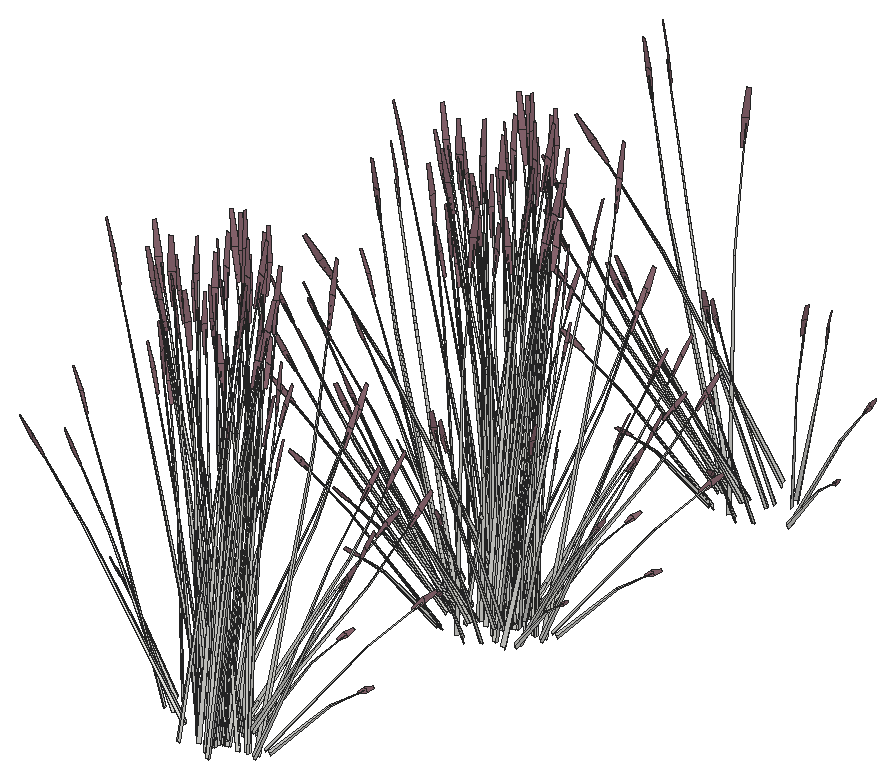
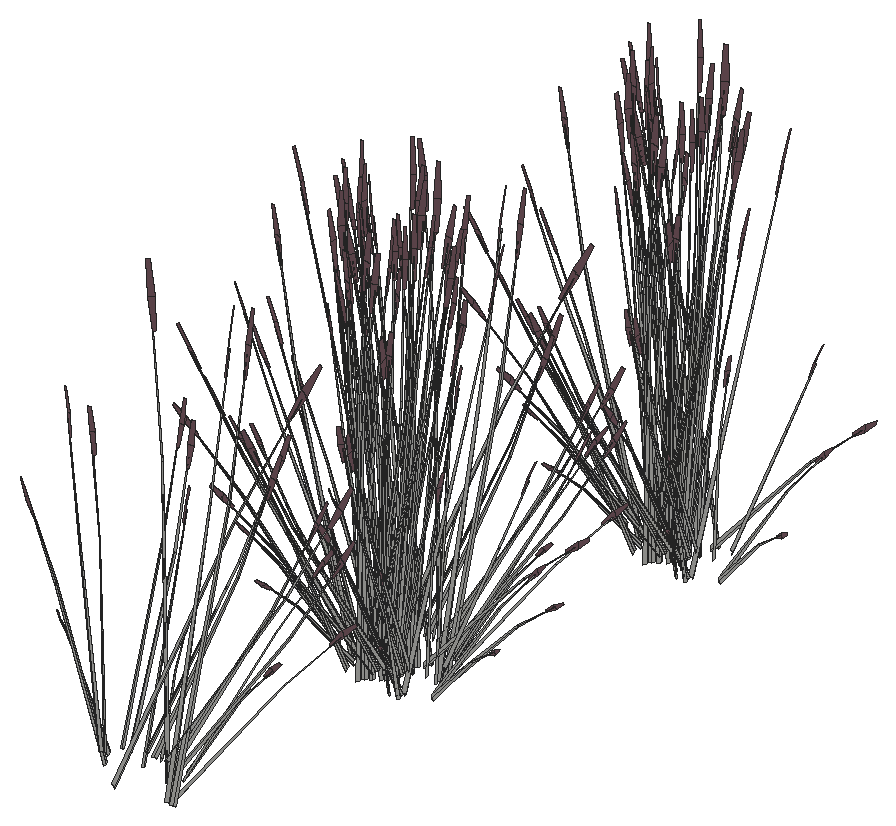
# SketchUp Ruby script. Lengths in inches.
U = 1.inch
M = Sketchup.active_model
def pt(a) = Geom::Point3d.new(a.map { |v| v * U })
def face(e, loops, mat)
  f = e.add_face(loops[0].map { |a| pt(a) })
  loops[1..].each { |l| e.add_face(l.map { |a| pt(a) }).erase! }
  f.material = f.back_material = mat if mat
  f
end
# faces: each face lists its corners as indices into pts; further lists are holes
def faces(e, pts, list, mat = nil) = list.each { |f| face(e, (f[0].is_a?(Array) ? f : [f]).map { |l| l.map { |i| pts[i] } }, mat) }
# xy, xz, yz: faces in a plane at the given z, y or x. An outline is a flat list of corners, or four numbers for a rectangle; further outlines are holes
def ring(l) = l.size == 4 ? [[l[0], l[1]], [l[2], l[1]], [l[2], l[3]], [l[0], l[3]]] : l.each_slice(2).to_a
def flat(e, list, mat, &to3) = list.each { |f| face(e, (f[0].is_a?(Array) ? f : [f]).map { |l| ring(l).map { |u, v| to3.(u, v) } }, mat) }
def xy(e, z, list, mat = nil) = flat(e, list, mat) { |x, y| [x, y, z] }
def xz(e, y, list, mat = nil) = flat(e, list, mat) { |x, z| [x, y, z] }
def yz(e, x, list, mat = nil) = flat(e, list, mat) { |y, z| [x, y, z] }
def lines(e, pts, list) = list.each { |a, b| e.add_line(pt(pts[a]), pt(pts[b])) }
# prism: a flat outline (further loops are holes) pulled along v
def prism(e, loops, v, mat = nil)
  f = face(e, loops, mat); d = Geom::Vector3d.new(v.map { |x| x * U })
  f.pushpull(f.normal.samedirection?(d) ? d.length : -d.length)
end
def box(e, o, s, mat = nil) = prism(e, [[o, [o[0] + s[0], o[1], o[2]], [o[0] + s[0], o[1] + s[1], o[2]], [o[0], o[1] + s[1], o[2]]]], [0, 0, s[2]], mat)
def at(x, y, z, deg = 0) = Geom::Transformation.translation(pt([x, y, z])) * Geom::Transformation.rotation(ORIGIN, Z_AXIS, deg.degrees)
def axes(o, x, y, z) = Geom::Transformation.new([*x, 0, *y, 0, *z, 0, *pt(o).to_a, 1])
def part(name) = M.definitions.add(name)
# library, detail: a bought-in or finely detailed component or shape, given as its bounding box
def library(name, o, s) = part(name).tap { |d| box(d.entities, o, s) }
def detail(e, o, s) = box(e.add_group.entities, o, s)
def put(e, d, t, mat = nil) = e.add_instance(d, t).tap { |i| i.material = mat if mat }
def group(e, t, mat = nil) = e.add_group.tap { |g| g.transformation = t; g.material = mat if mat }.entities
root = M.entities
M.materials.add("LightPink_Translucent").color = [144, 107, 117]
c1 = part("blade")
p = [[2.15,0.21,22],[0,0.17,0],[0.09,0.45,0],[2.18,0.31,22],[2.29,0.31,22],[0.38,0.45,0],
  [2.48,0.24,33],[2.49,0.24,33],[2.48,0.22,33]]
faces(c1.entities,p,[[0,1,2,3],[4,5,2,3],[6,3,4,7],[8,0,3,6]])
c2 = part("seeds")
p = [[0.3,-0.1,1.38],[-0.01,-0.03,1.59],[-0.01,-0.03,0.03],[0.14,-0.07,-0.07],[0.29,-0.03,3],[0.15,0.01,3.11]]
faces(c2.entities,p,[[0,1,2,3],[1,0,4,5]],"LightPink_Translucent")
c3 = part("blade with seeds")
put(c3.entities,c1,at(0,0,0))
put(c3.entities,c2,axes([2.4,0.25,30.99],[1.5799,-0.05474,1.17369],[-0.12525,1.92788,0.29478],[-0.07173,-0.02425,1.56792]))
put(root,c3,axes([33.5,392.59,44.36],[0.53281,1.15808,0.45755],[-1.52239,0.4027,0.17955],[0.01861,-0.2128,1.58856]))
put(root,c3,axes([40.95,393.48,43.98],[-0.7893,0.12429,1.41583],[-0.12563,-0.9893,0.08104],[0.55282,-0.14974,0.80566]))
put(root,c3,axes([33.24,393.5,44.72],[-0.59459,0.93321,0.44739],[-1.23546,-0.44912,-0.21531],[0,-0.21512,1.43643]))
put(root,c3,axes([35.42,392.69,44.21],[0,-1.19833,0],[1.53239,0,0],[0,0,1.79456]))
put(root,c3,axes([37.28,389.92,44.48],[-1.14694,-0.51783,0.49651],[0.68554,-0.92854,0],[0.26122,0.11794,1.57504]))
put(root,c3,axes([39.52,393.56,46.98],[1.07686,-0.45739,-0.71045],[0.60013,0.94154,0.08574],[0.52031,-0.10696,1.00501]))
put(root,c3,axes([34.69,391.93,44.36],[-1.01611,0.93987,0.45755],[-1.20717,-0.82966,0.17955],[0.24496,-0.0938,1.58856]))
put(root,c3,axes([35.8,393.62,44.3],[-1.1399,-0.8914,-0.06131],[1.1406,-0.89194,0],[-0.03981,-0.03113,1.75571]))
put(root,c3,axes([32.93,390.39,44.47],[-0.35402,1.02926,0.17642],[-1.29548,-0.29127,0.35086],[0.22379,-0.00501,1.60407]))
put(root,c3,axes([35.64,391.53,44.62],[0.23642,-0.92427,0.1448],[1.15506,0.16044,-0.41347],[0.21021,0.09491,1.26744]))
put(root,c3,axes([33.64,393.73,44.36],[1.54892,0.2182,0.45755],[-0.31522,1.23236,0.17955],[-0.22636,-0.119,1.58856]))
put(root,c3,axes([35.14,391.77,44.72],[-0.73619,-0.86927,0.44739],[1.11511,-0.61213,-0.21531],[0.23824,0.10756,1.43643]))
put(root,c3,axes([32.8,395.7,44.47],[1.31687,-0.27488,0.17642],[0.32517,1.02297,0.35086],[-0.11745,-0.14905,1.60407]))
put(root,c3,axes([36.46,392.96,44.21],[1.37109,0,0],[0,1.07219,0],[0,0,1.78407]))
put(root,c3,axes([36.85,390.44,44.47],[-1.31687,0.27488,0.17642],[-0.32517,-1.02297,0.35086],[0.11745,0.14905,1.60407]))
put(root,c3,axes([36.02,392.41,44.38],[-1.54892,-0.2182,0.49198],[0.31522,-1.23236,0.19306],[0.22636,0.119,1.70813]))
put(root,c3,axes([34.78,395.45,44.2],[-0.39985,-0.89288,0],[1.1418,-0.31268,0],[0,0,1.54371]))
put(root,c3,axes([34.02,394.61,44.62],[-0.23642,0.92427,0.1448],[-1.15506,-0.16044,-0.41347],[-0.21021,-0.09491,1.26744]))
put(root,c3,axes([36.72,395.75,44.47],[0.35402,-1.02926,0.17642],[1.29548,0.29127,0.35086],[-0.22379,0.00501,1.60407]))
put(root,c3,axes([36.43,393.42,44.21],[0.85545,0.66896,0],[-0.85545,0.66896,0],[0,0,1.69266]))
put(root,c3,axes([31.57,392.16,45.34],[0.34834,-0.14982,1.77064],[0.12012,1.04605,0.13857],[-0.75452,0.1388,0.63284]))
put(root,c3,axes([38.75,393.125,44.47],[-0.96285,-0.75439,0.17642],[0.97031,-0.7317,0.35086],[-0.10634,0.15406,1.60407]))
put(root,c3,axes([42.6,393.82,44.77],[-0.75718,0.17097,1.1486],[0.35641,-0.70661,0.84392],[0.40168,0.04835,0.25299]))
put(root,c3,axes([34.5,395.86,44.2],[-1.23546,-0.46496,0],[0.59459,-0.96613,0],[0,0,1.62707]))
put(root,c3,axes([32.375,396.22,44.48],[1.14694,0.51783,0.49651],[-0.68554,0.92854,0],[-0.26122,-0.11794,1.57504]))
put(root,c3,axes([36.42,392.63,44.72],[0.59459,-0.93321,0.44739],[1.23546,0.44912,-0.21531],[0,0.21512,1.43643]))
put(root,c3,axes([36.19,393.17,44.29],[0,1.19774,-0.05637],[-1.53239,0,0],[0,0.03764,1.79368]))
put(root,c3,axes([29.16,392.73,46.68],[-0.332,0.94205,-0.51099],[-1.13828,-0.3229,-0.3958],[-0.45829,0.08638,0.97773]))
put(root,c3,axes([31.72,396.76,44.375],[-0.7662,1.03778,0],[-1.28187,-0.57875,-0.51607],[-0.29196,-0.13181,1.63711]))
put(root,c3,axes([39.54,393.15,44.48],[0,-1.03566,0.49651],[1.37109,0,0],[0,0.23588,1.57504]))
put(root,c3,axes([36.1,393.93,44.72],[1.33077,-0.06393,0.44739],[0.12035,1.06125,-0.21531],[-0.23824,0.10756,1.43643]))
put(root,c3,axes([36.93,392.85,44.62],[1.1418,-0.30203,0.1448],[0.39985,0.86246,-0.41347],[0,0.18981,1.26744]))
put(root,c3,axes([41.18,394.95,44.59],[-0.29514,-0.25472,1.43002],[0.38401,-0.84262,-0.30754],[0.59714,0.11414,0.61141]))
put(root,c3,axes([35.9,395.875,44.2],[1.23546,0.46496,0],[-0.59459,0.96613,0],[0,0,1.74954]))
put(root,c3,axes([36.39,396.9,44.19],[-0.75665,-1.04141,-0.05142],[1.28187,-0.57875,0.51607],[-0.31588,0.09915,1.6363]))
put(root,c3,axes([36.125,394.39,44.62],[0.90538,0.62224,0.1448],[-0.75521,0.70202,-0.41347],[-0.21021,0.09491,1.26744]))
put(root,c3,axes([38.47,395.46,46.98],[1.22504,0.02494,-0.71045],[-0.08228,1.05005,0.08574],[0.51899,0.11081,1.00501]))
put(root,c3,axes([37.09,396.3,44.48],[1.14694,-0.51783,0.49651],[0.68554,0.92854,0],[-0.26122,0.11794,1.57504]))
put(root,c3,axes([35.46,395.49,44.29],[0.53281,1.18979,-0.06012],[-1.52239,0.41691,0],[0.01861,0.04155,1.72173]))
put(root,c3,axes([27.8,394.94,44.59],[0.42589,0.08502,1.43002],[0.2745,0.86839,-0.30754],[-0.57851,0.16255,0.61141]))
put(root,c3,axes([40.47,393.33,44.375],[1.53239,0,0],[0,1.1575,-0.51607],[0,0.26363,1.63711]))
put(root,c3,axes([39.86,393.93,44.2],[-1.53164,-0.00828,-0.04976],[0,-1.1575,0.49943],[-0.04813,0.2635,1.58352]))
put(root,c3,axes([26.91,396.76,44.77],[0.51072,-0.46938,1.1486],[0.20153,0.74307,0.84392],[-0.36908,0.13305,0.25299]))
put(root,c3,axes([36.43,396.37,44.33],[1.53422,0.33662,0.30756],[-0.38383,1.20322,-0.36492],[-0.25393,0.15059,1.64885]))
put(root,c3,axes([38.39,396.26,44.77],[-0.69001,-0.29779,1.1486],[0.89096,-0.30257,0.84392],[0.24031,0.2563,0.25299]))
put(root,c3,axes([29.72,394.83,46.68],[0.31482,0.94565,-0.51099],[-1.19224,0.16542,-0.3958],[-0.34166,0.254,0.97773]))
put(root,c3,axes([37.36,397.02,44.375],[0.7662,1.03778,0],[-1.28187,0.57875,-0.51607],[-0.29196,0.13181,1.63711]))
put(root,c3,axes([36.71,392.91,44.84],[-0.03348,-0.97511,1.41272],[1.51511,0.25277,0.59816],[-0.35835,0.53357,1.3335]))
put(root,c3,axes([36.83,396.67,46.68],[1.20928,-0.24619,-0.51099],[0.21154,0.93233,-0.3958],[0.32481,0.26718,0.97773]))
put(root,c3,axes([38.5,397.62,44.67],[-0.78586,-0.03248,1.0506],[0.51898,-0.68985,0.58006],[0.31045,0.24509,0.8241]))
put(root,c3,axes([35.93,395.95,44.59],[0.02163,-0.34331,1.43002],[1.03345,-0.38348,-0.30754],[0.31903,0.4109,0.61141]))
put(root,c3,axes([31.24,398.81,44.77],[-0.03171,-0.6158,1.1486],[0.7925,0.43922,0.84392],[-0.15586,0.29352,0.25299]))
put(root,c3,axes([31.54,396.43,47],[0.87728,0.69587,-0.5672],[-0.92674,0.60943,-0.43934],[-0.13348,0.35356,1.08528]))
put(root,c3,axes([30.59,397.48,44.82],[1.11329,-0.1834,0.06507],[0.25594,0.73887,-0.86304],[-0.07058,0.37403,0.7736]))
put(root,c3,axes([34.14,397.11,46.68],[1.20468,0.25962,-0.51099],[-0.41292,0.89013,-0.3958],[0.11046,0.35838,0.97773]))
put(root,c3,axes([31.27,396.11,47.34],[-0.03189,0.95798,-0.7886],[-1.34277,-0.06434,0.09517],[-0.14171,0.40585,1.11556]))
put(root,c3,axes([33.7,396.9375,46.98],[0.5849,0.8421,-0.71045],[-1.20401,0.4693,0.08574],[0.13677,0.40688,1.00501]))
put(root,c3,axes([30.32,398.26,44.59],[0.38672,-0.16338,1.43002],[0.95481,0.49262,-0.30754],[-0.28419,0.42626,0.61141]))
put(root,c3,axes([30.82,397.46,45.36],[0.02693,-0.53464,1.54345],[1.21102,0.2824,0.21329],[-0.10493,0.5698,0.72882]))
put(root,c3,axes([44.9375,427.97,44.59],[-0.34835,0.20963,1.43002],[-1.04325,-0.36691,-0.30754],[0.19338,-0.4563,0.61141]))
put(root,c3,axes([43.35,428.7,46.98],[-0.5849,-0.8421,-0.71045],[1.20401,-0.4693,0.08574],[-0.13677,-0.40688,1.00501]))
put(root,c3,axes([39.55,427.57,44.59],[-0.07421,0.33879,1.43002],[-1.08488,0.28361,-0.30754],[-0.25359,-0.4379,0.61141]))
put(root,c3,axes([45.79,429.52,46.98],[0.03189,-0.95798,-0.71045],[1.34277,0.06434,0.08574],[0.14171,-0.40585,1.00501]))
put(root,c3,axes([42.91,428.53,46.68],[-1.20468,-0.25962,-0.51099],[0.41292,-0.89013,-0.3958],[-0.11046,-0.35838,0.97773]))
put(root,c3,axes([43.66,426.3,44.77],[0.15721,0.60392,1.1486],[-0.87211,-0.33448,0.84392],[0.09385,-0.30923,0.25299]))
put(root,c3,axes([45.51,429.2,46.68],[-0.87728,-0.69587,-0.51099],[0.92674,-0.60943,-0.3958],[0.13348,-0.35356,0.97773]))
put(root,c3,axes([39.17,427.03,44.77],[0.63926,0.36046,1.1486],[-0.93099,0.21668,0.84392],[-0.1992,-0.27702,0.25299]))
put(root,c3,axes([40.72,428.9375,46.98],[-1.04497,-0.50058,-0.71045],[0.74264,-0.8772,0.08574],[-0.3786,-0.29889,1.00501]))
put(root,c3,axes([40.23,428.96,46.68],[-1.20928,0.24619,-0.51099],[-0.21154,-0.93233,-0.3958],[-0.32481,-0.26718,0.97773]))
put(root,c3,axes([47.37,431.1875,46.98],[0.64013,-0.81717,-0.71045],[1.12174,0.58074,0.08574],[0.38221,-0.29607,1.00501]))
put(root,c3,axes([40.45,428.81,44.375],[-0.7662,-1.03778,0],[1.28187,-0.57875,-0.51607],[0.29196,-0.13181,1.63711]))
put(root,c3,axes([47.34,430.81,46.68],[-0.31482,-0.94565,-0.51099],[1.19224,-0.16542,-0.3958],[0.34166,-0.254,0.97773]))
put(root,c3,axes([43.22,434.6,45.33],[1.05902,0.41762,1.51261],[-1.03748,0.89969,0.59816],[-0.46471,-0.53324,1.26806]))
put(root,c3,axes([48.3,430.4375,44.59],[-0.4378,-0.03068,1.43002],[-0.44851,-0.8229,-0.30754],[0.53783,-0.23279,0.61141]))
put(root,c3,axes([48.8,428.93,44.77],[-0.40819,0.5272,1.1486],[-0.35086,-0.70831,0.84392],[0.33713,-0.17749,0.25299]))
put(root,c3,axes([37.34,432.5,44.375],[-1.53239,0,0],[0,-1.1575,-0.51607],[0,-0.26363,1.63711]))
put(root,c3,axes([37.6,430.43,44.59],[0.23927,0.28834,1.43002],[-0.55135,0.78376,-0.30754],[-0.56612,-0.18733,0.61141]))
put(root,c3,axes([38.59,430.18,46.98],[-1.22504,-0.02494,-0.71045],[0.08228,-1.05005,0.08574],[-0.51899,-0.11081,1.00501]))
put(root,c3,axes([38.52,432.19,44.33],[-1.1399,0.87071,0.30756],[-1.1406,-0.86155,-0.36492],[-0.03981,-0.24727,1.64885]))
put(root,c3,axes([42.15,432.6,44.43],[1.3808,0.50196,0.24065],[-0.66454,1.04299,0.50002],[0,-0.24043,1.60543]))
put(root,c3,axes([38.18,430.39,46.68],[-0.88986,0.68603,-0.51099],[-0.77932,-0.72471,-0.3958],[-0.45212,-0.10438,0.97773]))
put(root,c3,axes([36.17,431.3,44.77],[0.78239,-0.07411,1.1486],[-0.49629,0.65296,0.84392],[-0.38663,-0.09795,0.25299]))
put(root,c3,axes([41.7,431.9,44.72],[-1.33077,0.06393,0.44739],[-0.12035,-1.06125,-0.21531],[0.23824,-0.10756,1.43643]))
put(root,c3,axes([38.27,432.68,44.48],[0,1.03566,0.49651],[-1.37109,0,0],[0,-0.23588,1.57504]))
put(root,c3,axes([47.89,432.91,46.68],[0.332,-0.94205,-0.51099],[1.13828,0.3229,-0.3958],[0.45829,-0.08638,0.97773]))
put(root,c3,axes([46.09,429.07,44.375],[0.7662,-1.03778,0],[1.28187,0.57875,-0.51607],[0.29196,0.13181,1.63711]))
put(root,c3,axes([41.66,432.28,44.36],[0.53281,1.15808,0.45755],[-1.52239,0.4027,0.17955],[0.01861,-0.2128,1.58856]))
put(root,c3,axes([49.11,433.17,43.98],[-0.7893,0.12429,1.41583],[-0.12563,-0.9893,0.08104],[0.55282,-0.14974,0.80566]))
put(root,c3,axes([41.39,433.2,44.72],[-0.59459,0.93321,0.44739],[-1.23546,-0.44912,-0.21531],[0,-0.21512,1.43643]))
put(root,c3,axes([43.57,432.38,44.21],[0,-1.19833,0],[1.53239,0,0],[0,0,1.79456]))
put(root,c3,axes([45.43,429.61,44.48],[-1.14694,-0.51783,0.49651],[0.68554,-0.92854,0],[0.26122,0.11794,1.57504]))
put(root,c3,axes([47.67,433.25,46.98],[1.07686,-0.45739,-0.71045],[0.60013,0.94154,0.08574],[0.52031,-0.10696,1.00501]))
put(root,c3,axes([42.85,431.625,44.36],[-1.01611,0.93987,0.45755],[-1.20717,-0.82966,0.17955],[0.24496,-0.0938,1.58856]))
put(root,c3,axes([43.96,433.31,44.3],[-1.1399,-0.8914,-0.06131],[1.1406,-0.89194,0],[-0.03981,-0.03113,1.75571]))
put(root,c3,axes([41.08,430.08,44.47],[-0.35402,1.02926,0.17642],[-1.29548,-0.29127,0.35086],[0.22379,-0.00501,1.60407]))
put(root,c3,axes([43.79,431.22,44.62],[0.23642,-0.92427,0.1448],[1.15506,0.16044,-0.41347],[0.21021,0.09491,1.26744]))
put(root,c3,axes([41.79,433.42,44.36],[1.54892,0.2182,0.45755],[-0.31522,1.23236,0.17955],[-0.22636,-0.119,1.58856]))
put(root,c3,axes([43.29,431.47,44.72],[-0.73619,-0.86927,0.44739],[1.11511,-0.61213,-0.21531],[0.23824,0.10756,1.43643]))
put(root,c3,axes([40.96,435.39,44.47],[1.31687,-0.27488,0.17642],[0.32517,1.02297,0.35086],[-0.11745,-0.14905,1.60407]))
put(root,c3,axes([44.61,432.65,44.21],[1.37109,0,0],[0,1.07219,0],[0,0,1.78407]))
put(root,c3,axes([45,430.14,44.47],[-1.31687,0.27488,0.17642],[-0.32517,-1.02297,0.35086],[0.11745,0.14905,1.60407]))
put(root,c3,axes([44.17,432.1,44.38],[-1.54892,-0.2182,0.49198],[0.31522,-1.23236,0.19306],[0.22636,0.119,1.70813]))
put(root,c3,axes([42.93,435.15,44.2],[-0.39985,-0.89288,0],[1.1418,-0.31268,0],[0,0,1.54371]))
put(root,c3,axes([42.17,434.3,44.62],[-0.23642,0.92427,0.1448],[-1.15506,-0.16044,-0.41347],[-0.21021,-0.09491,1.26744]))
put(root,c3,axes([44.875,435.44,44.47],[0.35402,-1.02926,0.17642],[1.29548,0.29127,0.35086],[-0.22379,0.00501,1.60407]))
put(root,c3,axes([44.58,433.11,44.21],[0.85545,0.66896,0],[-0.85545,0.66896,0],[0,0,1.69266]))
put(root,c3,axes([39.72,431.85,45.34],[0.34834,-0.14982,1.77064],[0.12012,1.04605,0.13857],[-0.75452,0.1388,0.63284]))
put(root,c3,axes([46.9,432.82,44.47],[-0.96285,-0.75439,0.17642],[0.97031,-0.7317,0.35086],[-0.10634,0.15406,1.60407]))
put(root,c3,axes([50.75,433.51,44.77],[-0.75718,0.17097,1.1486],[0.35641,-0.70661,0.84392],[0.40168,0.04835,0.25299]))
put(root,c3,axes([42.65,435.55,44.2],[-1.23546,-0.46496,0],[0.59459,-0.96613,0],[0,0,1.62707]))
put(root,c3,axes([40.53,435.91,44.48],[1.14694,0.51783,0.49651],[-0.68554,0.92854,0],[-0.26122,-0.11794,1.57504]))
put(root,c3,axes([44.57,432.33,44.72],[0.59459,-0.93321,0.44739],[1.23546,0.44912,-0.21531],[0,0.21512,1.43643]))
put(root,c3,axes([44.34,432.86,44.29],[0,1.19774,-0.05637],[-1.53239,0,0],[0,0.03764,1.79368]))
put(root,c3,axes([37.32,432.42,46.68],[-0.332,0.94205,-0.51099],[-1.13828,-0.3229,-0.3958],[-0.45829,0.08638,0.97773]))
put(root,c3,axes([39.87,436.45,44.375],[-0.7662,1.03778,0],[-1.28187,-0.57875,-0.51607],[-0.29196,-0.13181,1.63711]))
put(root,c3,axes([47.69,432.85,44.48],[0,-1.03566,0.49651],[1.37109,0,0],[0,0.23588,1.57504]))
put(root,c3,axes([44.26,433.62,44.72],[1.33077,-0.06393,0.44739],[0.12035,1.06125,-0.21531],[-0.23824,0.10756,1.43643]))
put(root,c3,axes([45.09,432.54,44.62],[1.1418,-0.30203,0.1448],[0.39985,0.86246,-0.41347],[0,0.18981,1.26744]))
put(root,c3,axes([49.33,434.64,44.59],[-0.29514,-0.25472,1.43002],[0.38401,-0.84262,-0.30754],[0.59714,0.11414,0.61141]))
put(root,c3,axes([44.05,435.57,44.2],[1.23546,0.46496,0],[-0.59459,0.96613,0],[0,0,1.74954]))
put(root,c3,axes([44.55,436.6,44.19],[-0.75665,-1.04141,-0.05142],[1.28187,-0.57875,0.51607],[-0.31588,0.09915,1.6363]))
put(root,c3,axes([44.28,434.08,44.62],[0.90538,0.62224,0.1448],[-0.75521,0.70202,-0.41347],[-0.21021,0.09491,1.26744]))
put(root,c3,axes([46.62,435.15,46.98],[1.22504,0.02494,-0.71045],[-0.08228,1.05005,0.08574],[0.51899,0.11081,1.00501]))
put(root,c3,axes([45.24,436,44.48],[1.14694,-0.51783,0.49651],[0.68554,0.92854,0],[-0.26122,0.11794,1.57504]))
put(root,c3,axes([43.61,435.18,44.29],[0.53281,1.18979,-0.06012],[-1.52239,0.41691,0],[0.01861,0.04155,1.72173]))
put(root,c3,axes([35.95,434.63,44.59],[0.42589,0.08502,1.43002],[0.2745,0.86839,-0.30754],[-0.57851,0.16255,0.61141]))
put(root,c3,axes([48.62,433.02,44.375],[1.53239,0,0],[0,1.1575,-0.51607],[0,0.26363,1.63711]))
put(root,c3,axes([48.01,433.62,44.2],[-1.53164,-0.00828,-0.04976],[0,-1.1575,0.49943],[-0.04813,0.2635,1.58352]))
put(root,c3,axes([35.0625,436.45,44.77],[0.51072,-0.46938,1.1486],[0.20153,0.74307,0.84392],[-0.36908,0.13305,0.25299]))
put(root,c3,axes([44.58,436.0625,44.33],[1.53422,0.33662,0.30756],[-0.38383,1.20322,-0.36492],[-0.25393,0.15059,1.64885]))
put(root,c3,axes([46.54,435.96,44.77],[-0.69001,-0.29779,1.1486],[0.89096,-0.30257,0.84392],[0.24031,0.2563,0.25299]))
put(root,c3,axes([37.87,434.52,46.68],[0.31482,0.94565,-0.51099],[-1.19224,0.16542,-0.3958],[-0.34166,0.254,0.97773]))
put(root,c3,axes([45.51,436.71,44.375],[0.7662,1.03778,0],[-1.28187,0.57875,-0.51607],[-0.29196,0.13181,1.63711]))
put(root,c3,axes([44.86,432.61,44.84],[-0.03348,-0.97511,1.41272],[1.51511,0.25277,0.59816],[-0.35835,0.53357,1.3335]))
put(root,c3,axes([44.98,436.37,46.68],[1.20928,-0.24619,-0.51099],[0.21154,0.93233,-0.3958],[0.32481,0.26718,0.97773]))
put(root,c3,axes([46.65,437.3125,44.67],[-0.78586,-0.03248,1.0506],[0.51898,-0.68985,0.58006],[0.31045,0.24509,0.8241]))
put(root,c3,axes([44.08,435.64,44.59],[0.02163,-0.34331,1.43002],[1.03345,-0.38348,-0.30754],[0.31903,0.4109,0.61141]))
put(root,c3,axes([39.4,438.5,44.77],[-0.03171,-0.6158,1.1486],[0.7925,0.43922,0.84392],[-0.15586,0.29352,0.25299]))
put(root,c3,axes([39.69,436.125,47],[0.87728,0.69587,-0.5672],[-0.92674,0.60943,-0.43934],[-0.13348,0.35356,1.08528]))
put(root,c3,axes([38.74,437.17,44.82],[1.11329,-0.1834,0.06507],[0.25594,0.73887,-0.86304],[-0.07058,0.37403,0.7736]))
put(root,c3,axes([42.29,436.8,46.68],[1.20468,0.25962,-0.51099],[-0.41292,0.89013,-0.3958],[0.11046,0.35838,0.97773]))
put(root,c3,axes([39.42,435.81,47.34],[-0.03189,0.95798,-0.7886],[-1.34277,-0.06434,0.09517],[-0.14171,0.40585,1.11556]))
put(root,c3,axes([41.86,436.63,46.98],[0.5849,0.8421,-0.71045],[-1.20401,0.4693,0.08574],[0.13677,0.40688,1.00501]))
put(root,c3,axes([38.47,437.96,44.59],[0.38672,-0.16338,1.43002],[0.95481,0.49262,-0.30754],[-0.28419,0.42626,0.61141]))
put(root,c3,axes([38.97,437.16,45.36],[0.02693,-0.53464,1.54345],[1.21102,0.2824,0.21329],[-0.10493,0.5698,0.72882]))
put(root,c3,axes([51.29,467.24,44.59],[-0.34835,0.20963,1.43002],[-1.04325,-0.36691,-0.30754],[0.19338,-0.4563,0.61141]))
put(root,c3,axes([49.71,467.96,46.98],[-0.5849,-0.8421,-0.71045],[1.20401,-0.4693,0.08574],[-0.13677,-0.40688,1.00501]))
put(root,c3,axes([45.9,466.84,44.59],[-0.07421,0.33879,1.43002],[-1.08488,0.28361,-0.30754],[-0.25359,-0.4379,0.61141]))
put(root,c3,axes([52.14,468.79,46.98],[0.03189,-0.95798,-0.71045],[1.34277,0.06434,0.08574],[0.14171,-0.40585,1.00501]))
put(root,c3,axes([49.27,467.8,46.68],[-1.20468,-0.25962,-0.51099],[0.41292,-0.89013,-0.3958],[-0.11046,-0.35838,0.97773]))
put(root,c3,axes([50.01,465.57,44.77],[0.15721,0.60392,1.1486],[-0.87211,-0.33448,0.84392],[0.09385,-0.30923,0.25299]))
put(root,c3,axes([51.87,468.47,46.68],[-0.87728,-0.69587,-0.51099],[0.92674,-0.60943,-0.3958],[0.13348,-0.35356,0.97773]))
put(root,c3,axes([45.53,466.29,44.77],[0.63926,0.36046,1.1486],[-0.93099,0.21668,0.84392],[-0.1992,-0.27702,0.25299]))
put(root,c3,axes([47.07,468.2,46.98],[-1.04497,-0.50058,-0.71045],[0.74264,-0.8772,0.08574],[-0.3786,-0.29889,1.00501]))
put(root,c3,axes([46.58,468.23,46.68],[-1.20928,0.24619,-0.51099],[-0.21154,-0.93233,-0.3958],[-0.32481,-0.26718,0.97773]))
put(root,c3,axes([53.72,470.45,46.98],[0.64013,-0.81717,-0.71045],[1.12174,0.58074,0.08574],[0.38221,-0.29607,1.00501]))
put(root,c3,axes([46.8,468.07,44.375],[-0.7662,-1.03778,0],[1.28187,-0.57875,-0.51607],[0.29196,-0.13181,1.63711]))
put(root,c3,axes([53.69,470.07,46.68],[-0.31482,-0.94565,-0.51099],[1.19224,-0.16542,-0.3958],[0.34166,-0.254,0.97773]))
put(root,c3,axes([49.57,473.87,45.33],[1.05902,0.41762,1.51261],[-1.03748,0.89969,0.59816],[-0.46471,-0.53324,1.26806]))
put(root,c3,axes([54.65,469.7,44.59],[-0.4378,-0.03068,1.43002],[-0.44851,-0.8229,-0.30754],[0.53783,-0.23279,0.61141]))
put(root,c3,axes([55.16,468.19,44.77],[-0.40819,0.5272,1.1486],[-0.35086,-0.70831,0.84392],[0.33713,-0.17749,0.25299]))
put(root,c3,axes([43.69,471.76,44.375],[-1.53239,0,0],[0,-1.1575,-0.51607],[0,-0.26363,1.63711]))
put(root,c3,axes([43.95,469.7,44.59],[0.23927,0.28834,1.43002],[-0.55135,0.78376,-0.30754],[-0.56612,-0.18733,0.61141]))
put(root,c3,axes([44.94,469.44,46.98],[-1.22504,-0.02494,-0.71045],[0.08228,-1.05005,0.08574],[-0.51899,-0.11081,1.00501]))
put(root,c3,axes([44.88,471.46,44.33],[-1.1399,0.87071,0.30756],[-1.1406,-0.86155,-0.36492],[-0.03981,-0.24727,1.64885]))
